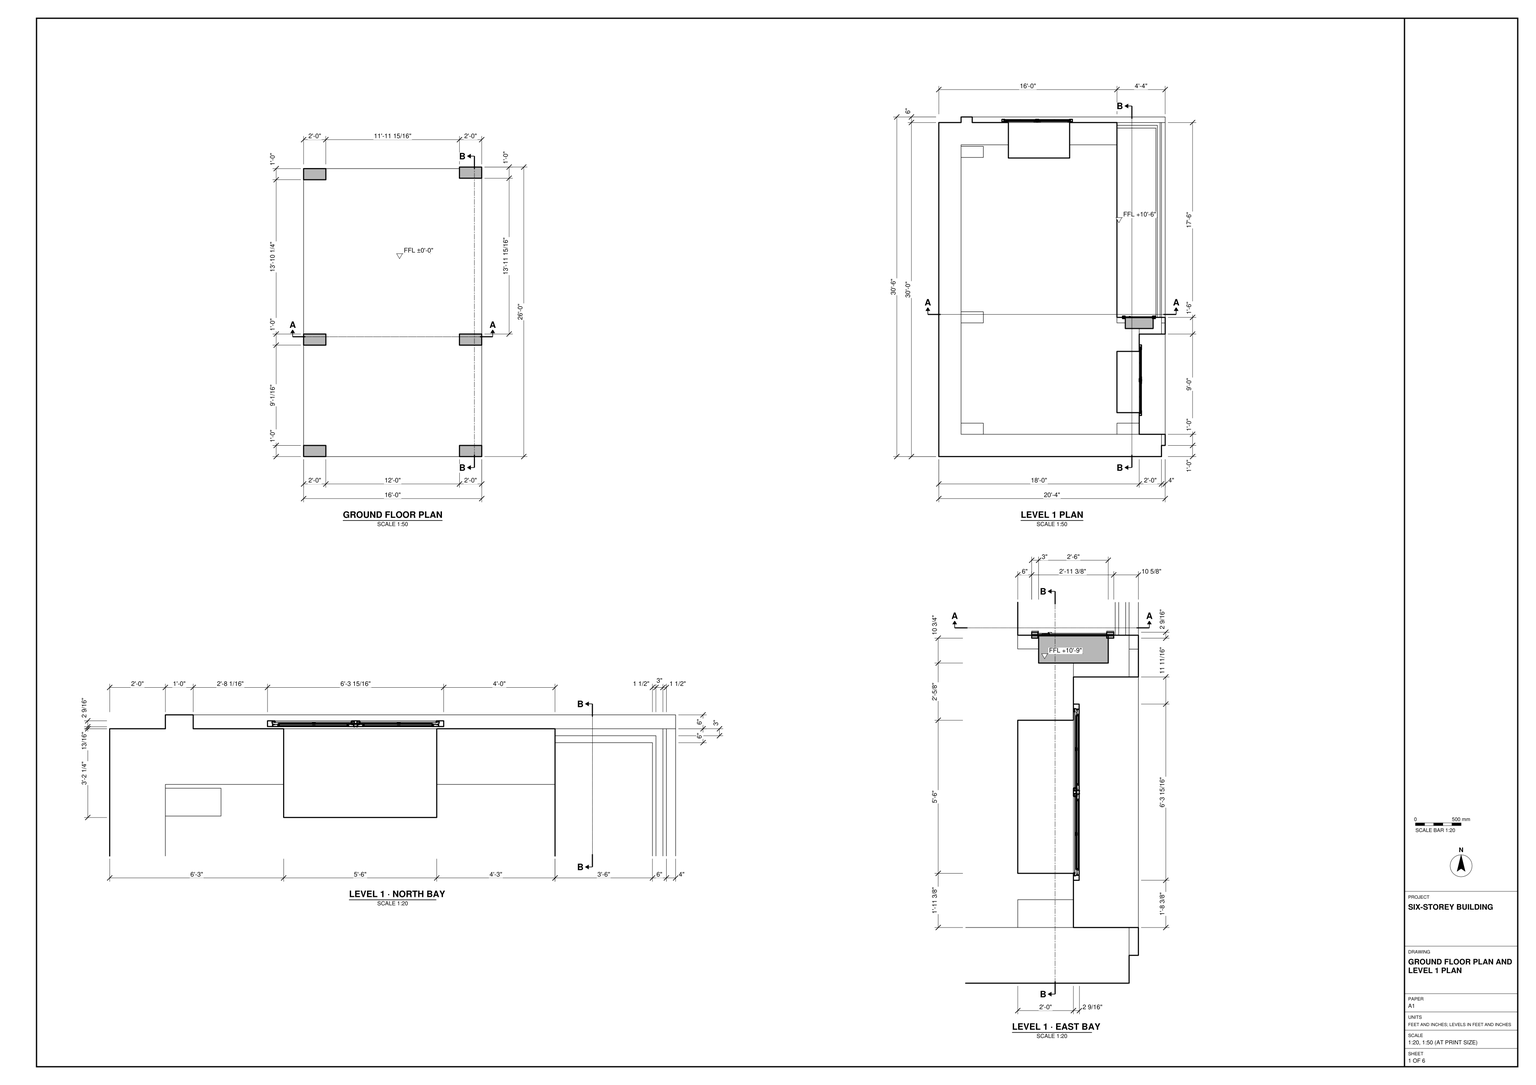
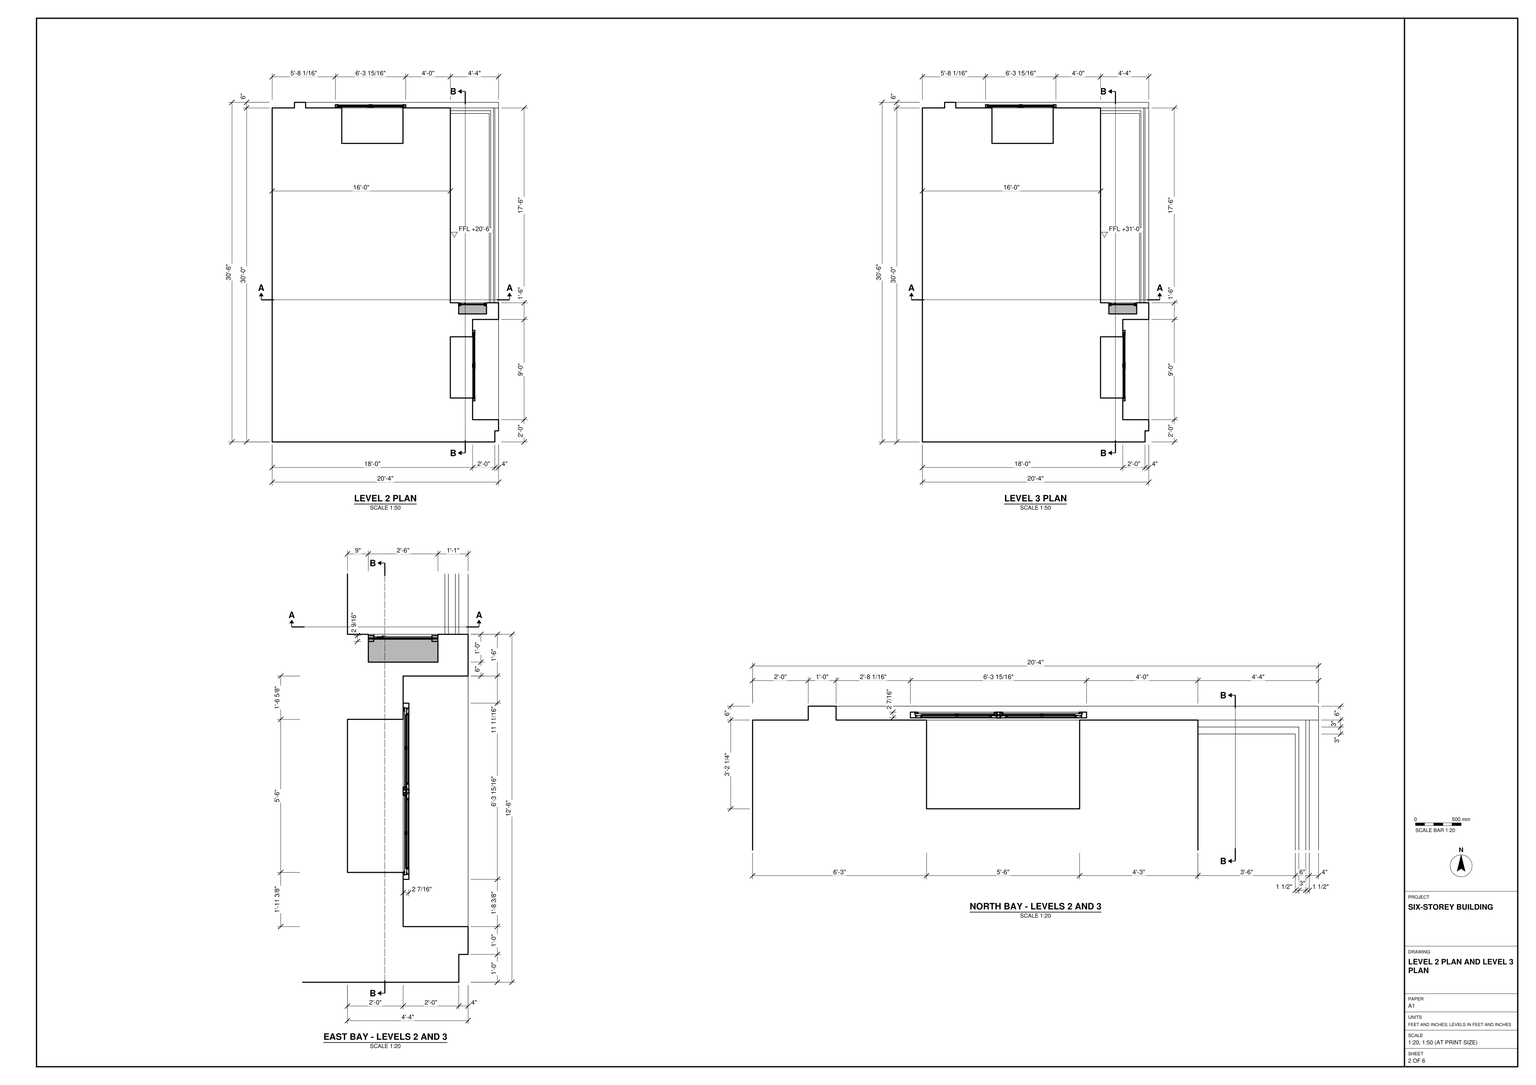
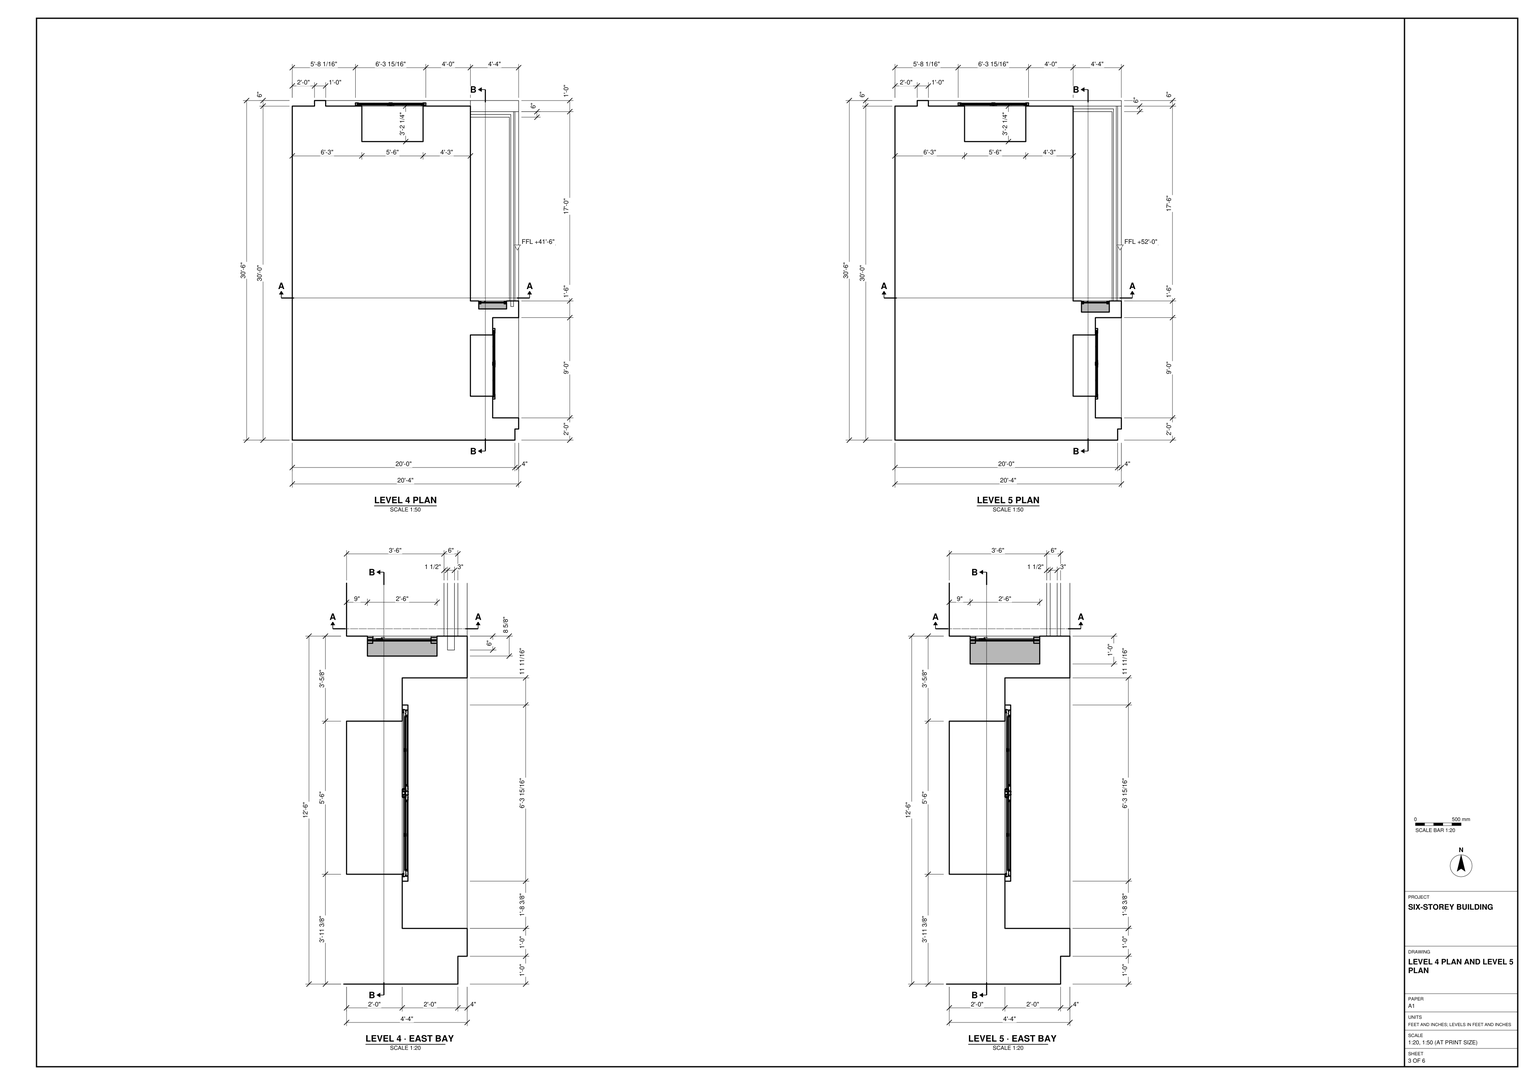
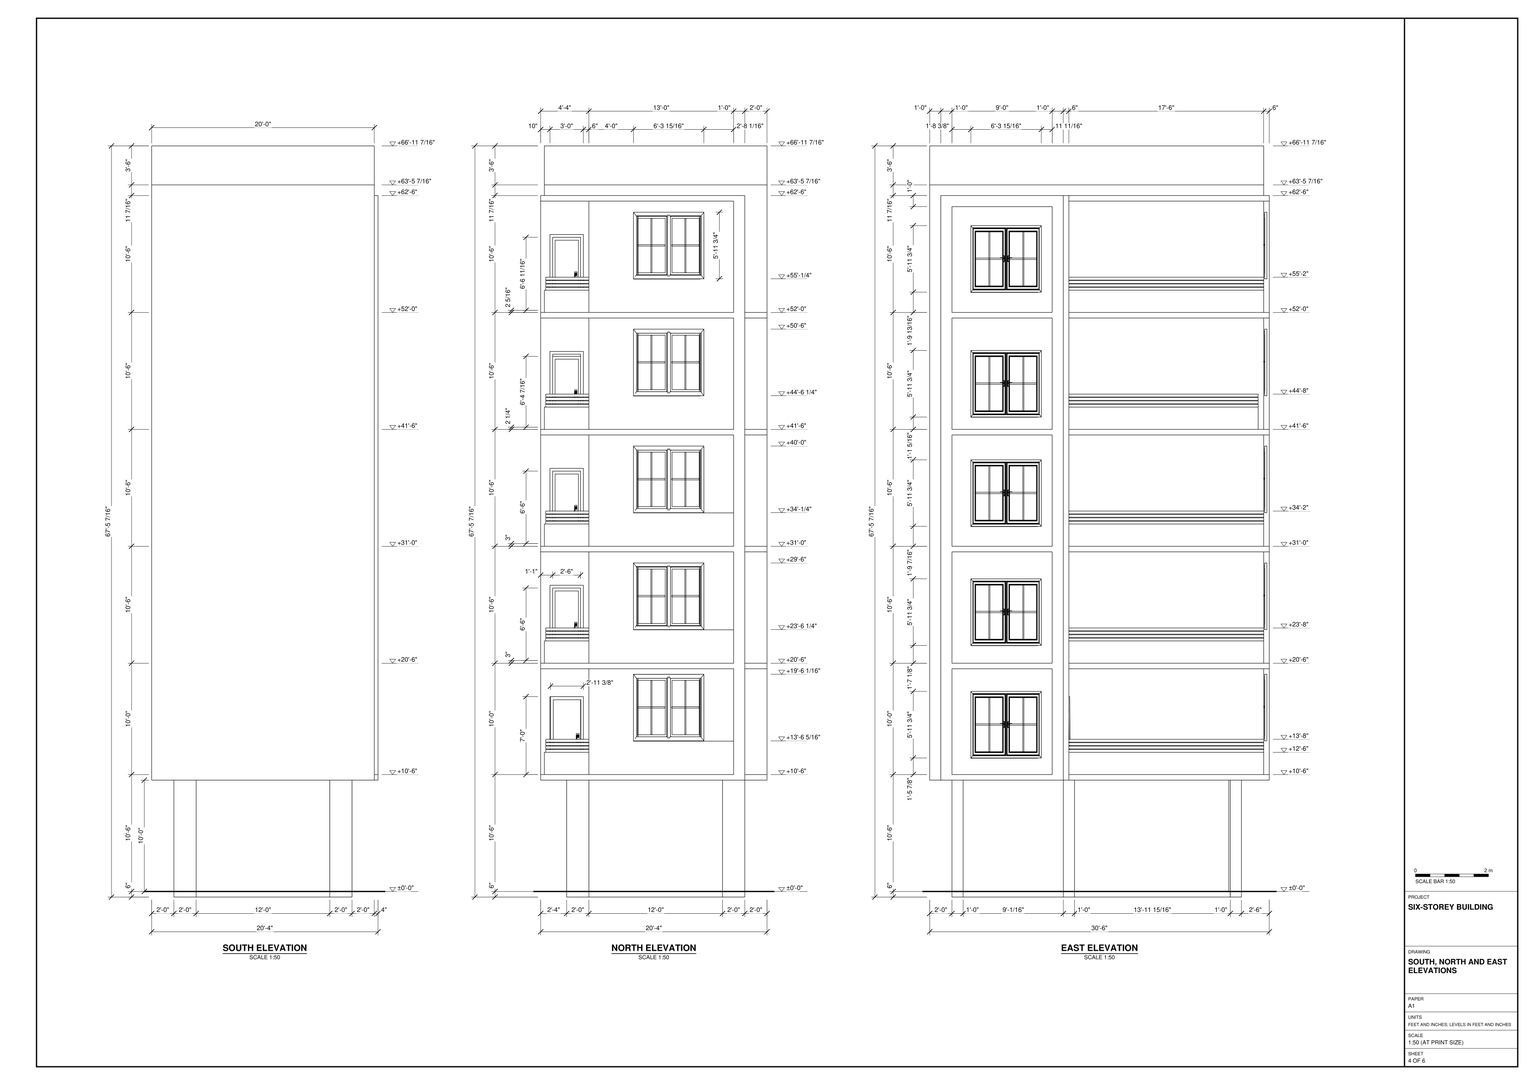
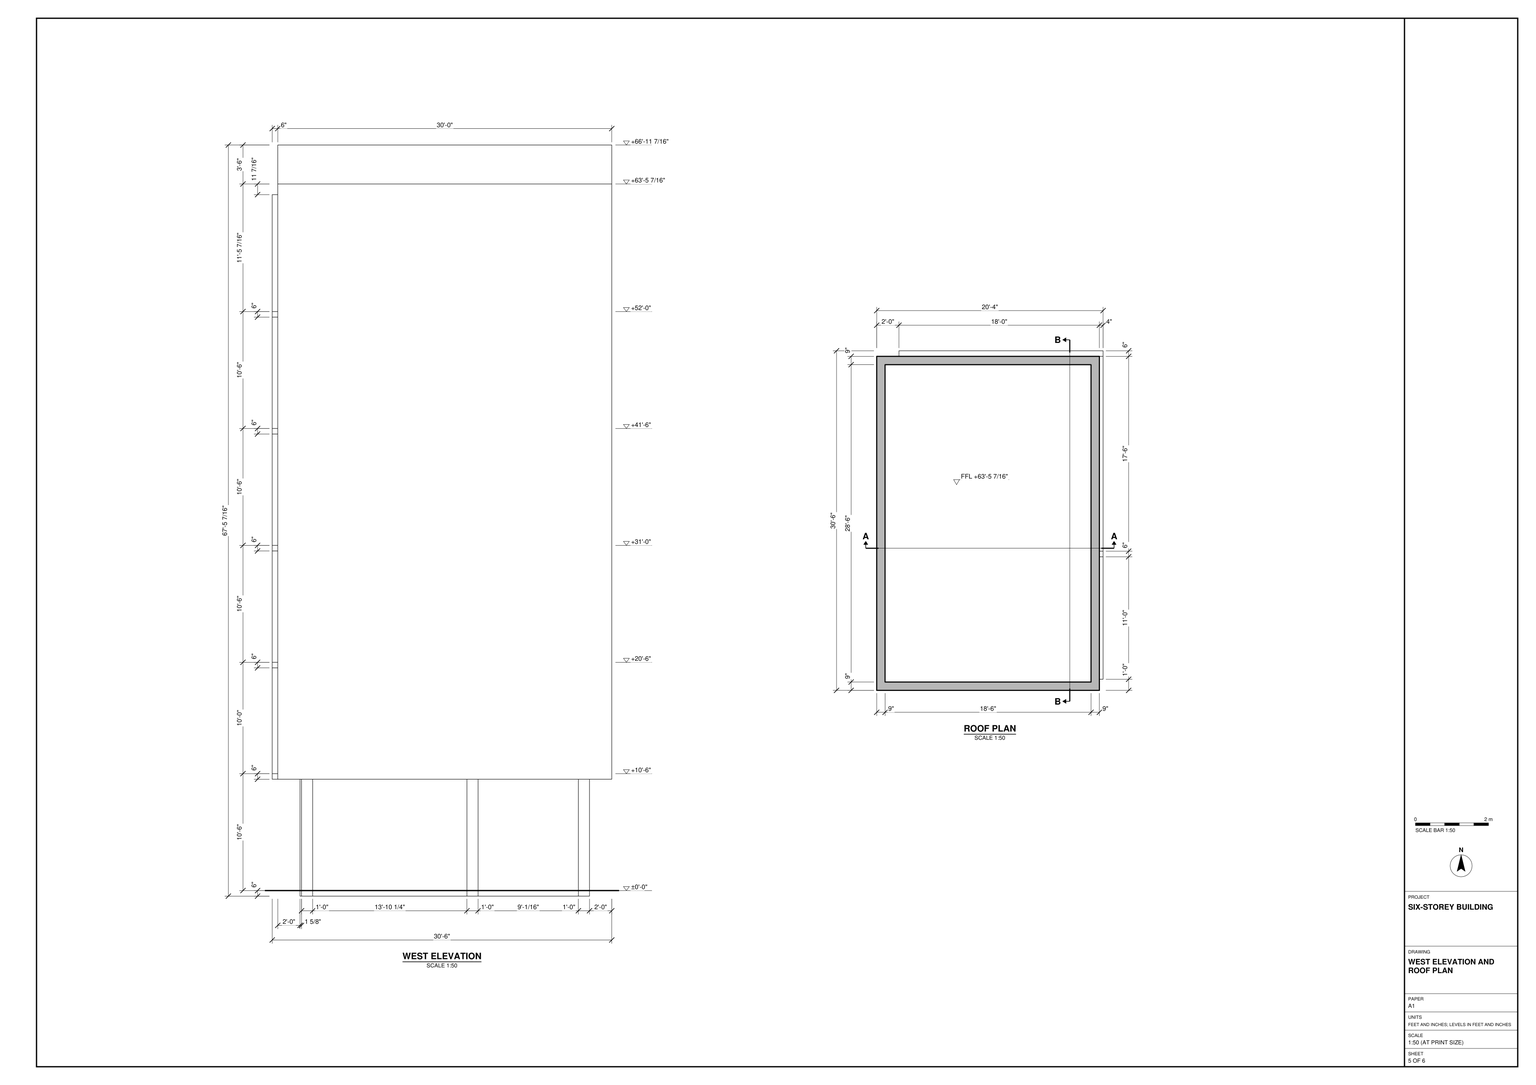
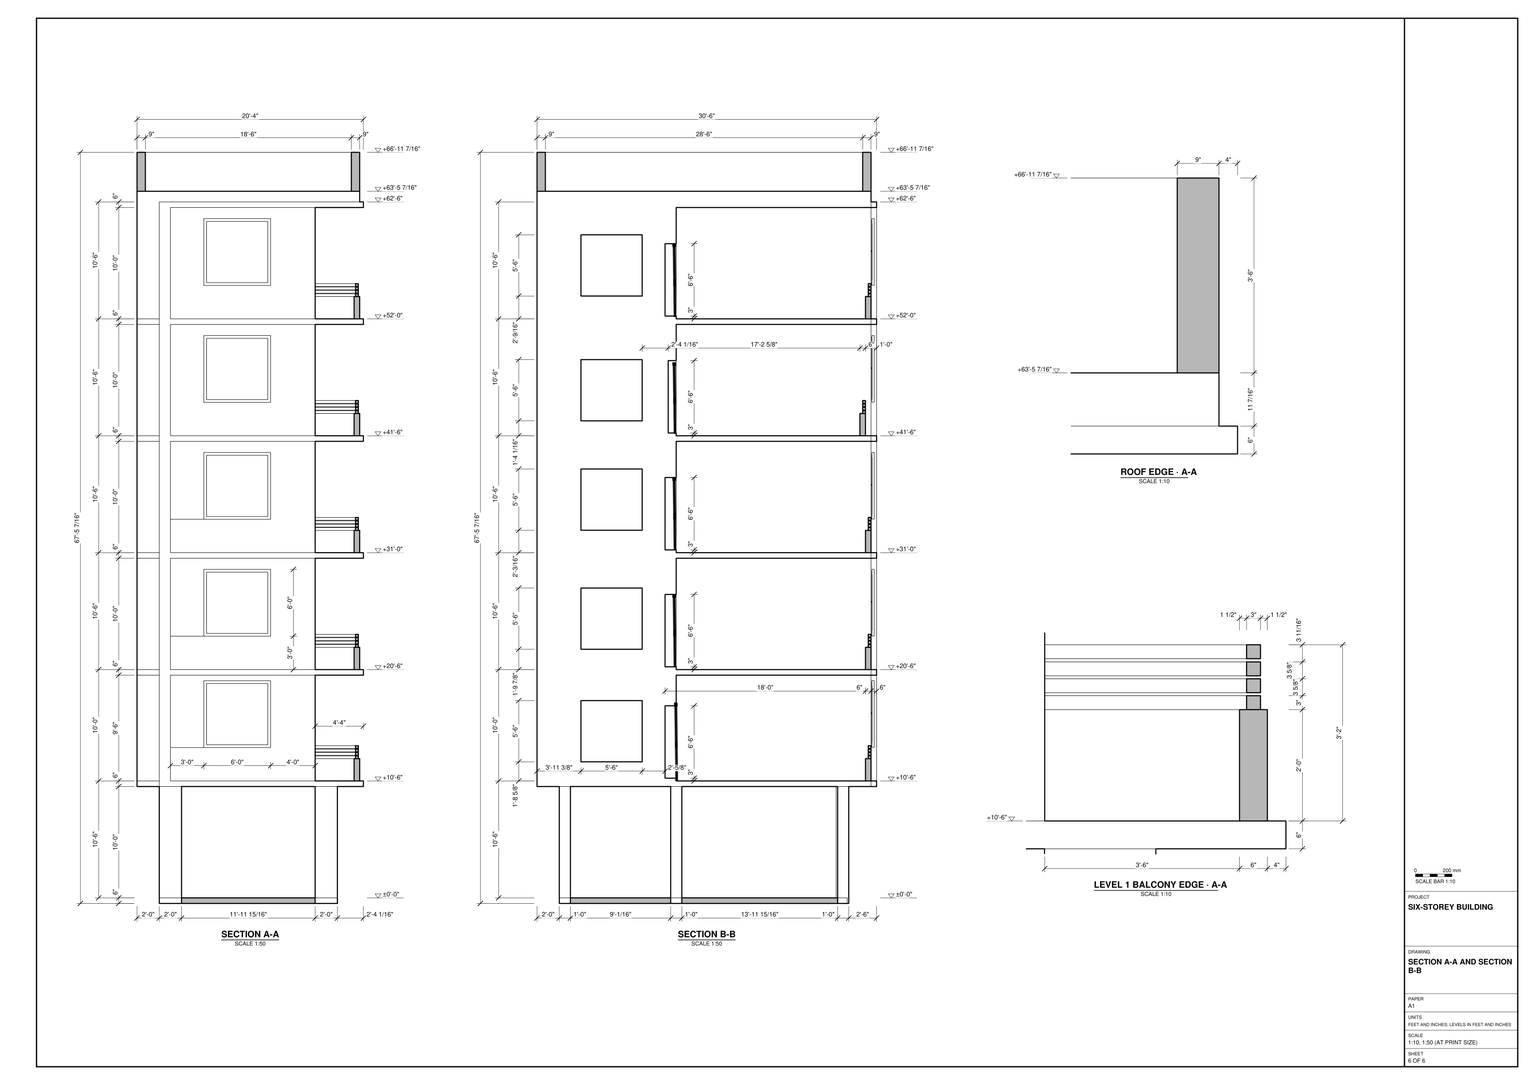
Build the six-storey building in SketchUp from task_files/diagram_01.pdf. Work in feet and inches. The overall size is 20'-4" east to west by 30'-6" north to south, with a total height of 67'-5 7/16". Set the ground floor at ±0'-0" and Levels 1 through 5 at +10'-6", +20'-6", +31'-0", +41'-6" and +52'-0", respectively.

Start with the two rows of rectangular ground-floor columns. Keep the ground storey open and position the upper slabs over the columns using the plans. Model the walls at their drawn thicknesses, the slab edges and the roof profile. On each upper floor, use the enlarged bay plans to locate the north opening, the long narrow bay at the northeast corner and the stepped east wall. Fit the door and window units into the openings, including the opening in the short return at the end of the narrow bay. Follow the detail for each level rather than assuming that every return is identical.

Keep walls, slabs and roof elements in separate groups or components. Group each furniture or joinery piece separately where shown, and use components for repeated parts. Any decor or loose items shown may be represented by suitable library components. Save one SketchUp model as output_files/six_storey_building_with_open_ground_floor.skp.

# SketchUp Ruby script. Lengths in inches.
U = 1.inch
M = Sketchup.active_model
def pt(a) = Geom::Point3d.new(a.map { |v| v * U })
def face(e, loops, mat)
  f = e.add_face(loops[0].map { |a| pt(a) })
  loops[1..].each { |l| e.add_face(l.map { |a| pt(a) }).erase! }
  f.material = f.back_material = mat if mat
  f
end
# faces: each face lists its corners as indices into pts; further lists are holes
def faces(e, pts, list, mat = nil) = list.each { |f| face(e, (f[0].is_a?(Array) ? f : [f]).map { |l| l.map { |i| pts[i] } }, mat) }
# xy, xz, yz: faces in a plane at the given z, y or x. An outline is a flat list of corners, or four numbers for a rectangle; further outlines are holes
def ring(l) = l.size == 4 ? [[l[0], l[1]], [l[2], l[1]], [l[2], l[3]], [l[0], l[3]]] : l.each_slice(2).to_a
def flat(e, list, mat, &to3) = list.each { |f| face(e, (f[0].is_a?(Array) ? f : [f]).map { |l| ring(l).map { |u, v| to3.(u, v) } }, mat) }
def xy(e, z, list, mat = nil) = flat(e, list, mat) { |x, y| [x, y, z] }
def xz(e, y, list, mat = nil) = flat(e, list, mat) { |x, z| [x, y, z] }
def yz(e, x, list, mat = nil) = flat(e, list, mat) { |y, z| [x, y, z] }
def lines(e, pts, list) = list.each { |a, b| e.add_line(pt(pts[a]), pt(pts[b])) }
# prism: a flat outline (further loops are holes) pulled along v
def prism(e, loops, v, mat = nil)
  f = face(e, loops, mat); d = Geom::Vector3d.new(v.map { |x| x * U })
  f.pushpull(f.normal.samedirection?(d) ? d.length : -d.length)
end
def box(e, o, s, mat = nil) = prism(e, [[o, [o[0] + s[0], o[1], o[2]], [o[0] + s[0], o[1] + s[1], o[2]], [o[0], o[1] + s[1], o[2]]]], [0, 0, s[2]], mat)
def at(x, y, z, deg = 0) = Geom::Transformation.translation(pt([x, y, z])) * Geom::Transformation.rotation(ORIGIN, Z_AXIS, deg.degrees)
def axes(o, x, y, z) = Geom::Transformation.new([*x, 0, *y, 0, *z, 0, *pt(o).to_a, 1])
def part(name) = M.definitions.add(name)
# library, detail: a bought-in or finely detailed component or shape, given as its bounding box
def library(name, o, s) = part(name).tap { |d| box(d.entities, o, s) }
def detail(e, o, s) = box(e.add_group.entities, o, s)
def put(e, d, t, mat = nil) = e.add_instance(d, t).tap { |i| i.material = mat if mat }
def group(e, t, mat = nil) = e.add_group.tap { |g| g.transformation = t; g.material = mat if mat }.entities
root = M.entities
M.materials.add("C01_Vanilla_Cream").color = [255, 230, 206]
M.materials.add("Carpet_04_1K").color = [43, 65, 85]
M.materials.add("M00_Soft_Cloud").color = [255, 255, 255]
M.materials.add("[Color_009]1").color = [0, 0, 0]
c1 = library("porta+4",[0.2,-5.42,1.33],[46.55,4.72,83.21])
c2 = library("mesh-163",[-551.08,-704.17,-20.03],[1929.24,1401.85,86.96])
c3 = part("Group11")
put(c3.entities,c2,at(0,0,0))
g1 = group(root,at(0,0,0))
xy(g1,-6,[[24,24,48,36],[[48,24,48,36,24,36,24,144.09,48,144.09,48,156.09,24,156.09,24,322.36,48,322.36,48,334.36,191.96,334.36,191.96,323.92,216,323.92,216,36,192,36,192,24],[191.96,144.09,215.96,156.09]],[192,24,216,36],[24,144.09,48,156.09],[191.96,144.09,215.96,156.09],
  [24,322.36,48,334.36],[191.96,324,215.96,336]])
xy(g1,0,[[[48,24,192,24,192,36,216,36,216,323.92,191.96,323.92,191.96,334.36,48,334.36,48,322.36,24,322.36,24,156.09,48,156.09,48,144.09,24,144.09,24,36,48,36],[191.96,144.09,215.96,156.09]]])
xy(g1,120,[[[0,0,0,360,24,360,24,366,36,366,36,360,240,360,240,0],[24,24,216,336]],[240,12,244,144],[[48,24,48,36,24,36,24,144.09,48,144.09,48,156.09,24,156.09,24,322.36,48,322.36,48,334.36,24,334.36,24,336,191.96,336,191.96,324,215.96,324,215.96,336,216,336,216,36,192,36,192,24],[191.96,144.09,215.96,156.09]],[240,144,244,360],[36,360,244,366]])
xy(g1,126,[[234,150,240,360],[192,354,234,360]])
xy(g1,126,[[216,24,244,132],[192,150,234,354],[240,150,244,360],[36,360,244,366]],"C01_Vanilla_Cream")
xy(g1,129,[[201,138,231,150]])
xy(g1,146.61,[[192,47.35,216,113.35]])
xy(g1,150,[[234,150,235.52,150,235.52,357,192,357,192,354,234,354],[235.52,150,235.52,357,192,357,192,360,238.52,360,238.52,150],[238.52,150,240,360]],"C01_Vanilla_Cream")
xy(g1,153,[[235.52,150,238.52,150,238.52,360,192,360,192,357,235.52,357]],"C01_Vanilla_Cream")
xy(g1,153.65,[[235.52,150,235.52,357,192,357,192,360,238.52,360,238.52,150]],"C01_Vanilla_Cream")
xy(g1,156.65,[[235.52,150,238.52,150,238.52,360,192,360,192,357,235.52,357]],"C01_Vanilla_Cream")
xy(g1,157.28,[[235.52,150,235.52,357,192,357,192,360,238.52,360,238.52,150]],"C01_Vanilla_Cream")
xy(g1,160.28,[[235.52,150,238.52,150,238.52,360,192,360,192,357,235.52,357]],"C01_Vanilla_Cream")
xy(g1,160.98,[[235.52,150,235.52,357,192,357,192,360,238.52,360,238.52,150]],"C01_Vanilla_Cream")
xy(g1,163.98,[[235.52,150,238.52,150,238.52,360,192,360,192,357,235.52,357]],"[Color_009]1")
xy(g1,165,[[75,321.76,141,360]])
xy(g1,207,[[201,138,231,150]])
xy(g1,212.61,[[192,47.35,216,113.35]])
xy(g1,231,[[75,321.76,141,360]])
xy(g1,240,[[216,24,244,132],[36,360,192,366]])
xy(g1,240,[[192,150,244,366]],"C01_Vanilla_Cream")
xy(g1,246,[[234,150,240,360],[192,354,234,360]])
xy(g1,246,[[216,24,244,132],[192,150,234,354],[240,150,244,360],[36,360,244,366]],"C01_Vanilla_Cream")
xy(g1,249,[[201,138,231,150]])
xy(g1,267.9,[[192,47.35,216,113.35]])
xy(g1,270,[[234,150,235.52,150,235.52,357,192,357,192,354,234,354],[235.52,150,235.52,357,192,357,192,360,238.52,360,238.52,150],[238.52,150,240,360]],"C01_Vanilla_Cream")
xy(g1,273,[[235.52,150,238.52,150,238.52,360,192,360,192,357,235.52,357]],"C01_Vanilla_Cream")
xy(g1,273.65,[[235.52,150,235.52,357,192,357,192,360,238.52,360,238.52,150]],"C01_Vanilla_Cream")
xy(g1,276.65,[[235.52,150,238.52,150,238.52,360,192,360,192,357,235.52,357]],"C01_Vanilla_Cream")
xy(g1,277.28,[[235.52,150,235.52,357,192,357,192,360,238.52,360,238.52,150]],"C01_Vanilla_Cream")
xy(g1,280.28,[[235.52,150,238.52,150,238.52,360,192,360,192,357,235.52,357]],"C01_Vanilla_Cream")
xy(g1,280.98,[[235.52,150,235.52,357,192,357,192,360,238.52,360,238.52,150]],"C01_Vanilla_Cream")
xy(g1,283.98,[[235.52,150,238.52,150,238.52,360,192,360,192,357,235.52,357]],"[Color_009]1")
xy(g1,285,[[75,321.76,141,360]])
xy(g1,327,[[201,138,231,150]])
xy(g1,333.9,[[192,47.35,216,113.35]])
xy(g1,351,[[75,321.76,141,360]])
xy(g1,366,[[216,24,244,132],[36,360,192,366]])
xy(g1,366,[[192,150,244,366]],"C01_Vanilla_Cream")
xy(g1,372,[[234,150,240,360],[192,354,234,360]])
xy(g1,372,[[216,24,244,132],[192,150,234,354],[240,150,244,360],[36,360,244,366]],"C01_Vanilla_Cream")
xy(g1,375,[[201,138,231,150]])
xy(g1,396,[[234,150,235.52,150,235.52,357,192,357,192,354,234,354],[235.52,150,235.52,357,192,357,192,360,238.52,360,238.52,150],[238.52,150,240,360]],"C01_Vanilla_Cream")
xy(g1,396.2,[[192,47.35,216,113.35]])
xy(g1,399,[[235.52,150,238.52,150,238.52,360,192,360,192,357,235.52,357]],"C01_Vanilla_Cream")
xy(g1,399.65,[[235.52,150,235.52,357,192,357,192,360,238.52,360,238.52,150]],"C01_Vanilla_Cream")
xy(g1,402.65,[[235.52,150,238.52,150,238.52,360,192,360,192,357,235.52,357]],"C01_Vanilla_Cream")
xy(g1,403.28,[[235.52,150,235.52,357,192,357,192,360,238.52,360,238.52,150]],"C01_Vanilla_Cream")
xy(g1,406.28,[[235.52,150,238.52,150,238.52,360,192,360,192,357,235.52,357]],"C01_Vanilla_Cream")
xy(g1,406.98,[[235.52,150,235.52,357,192,357,192,360,238.52,360,238.52,150]],"C01_Vanilla_Cream")
xy(g1,409.98,[[235.52,150,238.52,150,238.52,360,192,360,192,357,235.52,357]],"[Color_009]1")
xy(g1,411,[[75,321.76,141,360]])
xy(g1,453,[[201,138,231,150]])
xy(g1,462.2,[[192,47.35,216,113.35]])
xy(g1,477,[[75,321.76,141,360]])
xy(g1,492,[[36,360,192,366]])
xy(g1,492,[[216,24,244,132],[192,150,244,366]],"C01_Vanilla_Cream")
xy(g1,498,[[234,150,240,354],[192,348,234,354]])
xy(g1,498,[[216,24,244,132],[192,150,234,348],[240,150,244,354],[192,354,244,366],[36,360,192,366]],"C01_Vanilla_Cream")
xy(g1,501,[[201,141.4,231,150]])
xy(g1,514.07,[[192,47.35,216,113.35]])
xy(g1,522,[[235.52,144,238.52,150],[234,150,235.52,150,235.52,351,192,351,192,348,234,348],[235.52,150,238.52,150,238.52,354,192,354,192,351,235.52,351],[238.52,150,240,354]],"C01_Vanilla_Cream")
xy(g1,525,[[235.52,144,238.52,144,238.52,354,192,354,192,351,235.52,351]],"C01_Vanilla_Cream")
xy(g1,525.6,[[235.52,144,235.52,351,192,351,192,354,238.52,354,238.52,144]],"C01_Vanilla_Cream")
xy(g1,528.65,[[235.52,144,238.52,144,238.52,354,192,354,192,351,235.52,351]],"C01_Vanilla_Cream")
xy(g1,529.28,[[235.52,144,235.52,351,192,351,192,354,238.52,354,238.52,144]],"C01_Vanilla_Cream")
xy(g1,532.28,[[235.52,144,238.52,144,238.52,354,192,354,192,351,235.52,351]],"C01_Vanilla_Cream")
xy(g1,532.98,[[235.52,144,235.52,351,192,351,192,354,238.52,354,238.52,144]],"C01_Vanilla_Cream")
xy(g1,535.98,[[235.52,144,238.52,144,238.52,354,192,354,192,351,235.52,351]],"[Color_009]1")
xy(g1,537,[[75,321.76,141,360]])
xy(g1,579,[[201,141.4,231,150]])
xy(g1,580.07,[[192,47.35,216,113.35]])
xy(g1,603,[[75,321.76,141,360]])
xy(g1,618,[[36,360,192,366]])
xy(g1,618,[[216,24,244,132],[192,150,244,366]],"C01_Vanilla_Cream")
xy(g1,624,[[234,150,240,360],[192,354,234,360]])
xy(g1,624,[[216,24,244,132],[192,150,234,354],[240,150,244,360],[36,360,244,366]],"C01_Vanilla_Cream")
xy(g1,627,[[201,138,231,150]])
xy(g1,648,[[234,150,235.52,150,235.52,357,192,357,192,354,234,354],[235.52,150,238.52,150,238.52,360,192,360,192,357,235.52,357],[238.52,150,240,360]],"C01_Vanilla_Cream")
xy(g1,648.59,[[192,47.35,216,113.35]])
xy(g1,651,[[235.52,150,238.52,150,238.52,360,192,360,192,357,235.52,357]],"[Color_009]1")
xy(g1,651.65,[[235.52,150,235.52,357,192,357,192,360,238.52,360,238.52,150]],"C01_Vanilla_Cream")
xy(g1,654.65,[[235.52,150,238.52,150,238.52,360,192,360,192,357,235.52,357]],"[Color_009]1")
xy(g1,655.28,[[235.52,150,235.52,357,192,357,192,360,238.52,360,238.52,150]],"C01_Vanilla_Cream")
xy(g1,658.28,[[235.52,150,238.52,150,238.52,360,192,360,192,357,235.52,357]],"[Color_009]1")
xy(g1,658.98,[[235.52,150,235.52,357,192,357,192,360,238.52,360,238.52,150]],"C01_Vanilla_Cream")
xy(g1,661.98,[[235.52,150,238.52,150,238.52,360,192,360,192,357,235.52,357]],"[Color_009]1")
xy(g1,663,[[75,321.76,141,360]])
xy(g1,705,[[201,138,231,150]])
xy(g1,714.59,[[192,47.35,216,113.35]])
xy(g1,729,[[75,321.76,141,360]])
xy(g1,738,[[216,24,244,132]])
xy(g1,744,[[36,360,192,366]])
xy(g1,744,[[192,150,244,366]],"C01_Vanilla_Cream")
xy(g1,750,[[240,12,244,144],[240,144,244,150],[240,150,244,360],[24,360,244,366]],"C01_Vanilla_Cream")
xy(g1,761.46,[[9,9,231,351]],"C01_Vanilla_Cream")
xz(g1,0,[[0,120,240,761.46]],"C01_Vanilla_Cream")
xz(g1,12,[[240,120,244,126],[240,126,244,750]])
xz(g1,24,[[24,-6,48,120],[48,-6,192,0],[192,-6,216,120]])
xz(g1,24,[[216,126,244,240],[216,246,244,366],[216,372,244,492],[216,498,244,618],[216,624,244,738]],"C01_Vanilla_Cream")
xz(g1,36,[[24,-6,48,0],[192,-6,216,0],[24,0,48,120],[192,0,216,120]])
xz(g1,47.35,[[192,146.61,216,212.61],[192,267.9,216,333.9],[192,396.2,216,462.2],[192,514.07,216,580.07],[192,648.59,216,714.59]])
xz(g1,113.35,[[192,146.61,216,212.61],[192,267.9,216,333.9],[192,396.2,216,462.2],[192,514.07,216,580.07],[192,648.59,216,714.59]])
xz(g1,132,[[216,126,244,240],[216,246,244,366],[216,372,244,492],[216,498,244,618],[216,624,244,738]],"C01_Vanilla_Cream")
xz(g1,138,[[201,129,231,207],[201,249,231,327],[201,375,231,453],[201,627,231,705]])
xz(g1,141.4,[[201,501,231,579]])
xz(g1,144,[[235.52,522,238.52,525],[235.52,525.6,238.52,528.65],[235.52,529.28,238.52,532.28],[235.52,532.98,238.52,535.98]],"C01_Vanilla_Cream")
xz(g1,144.09,[[24,-6,48,0],[191.96,-6,215.96,0],[24,0,48,120],[191.96,0,215.96,120]])
xz(g1,150,[[[198,126,234,210],[201,129,231,207]],[234,126,240,150],[[198,246,234,330],[201,249,231,327]],[234,246,240,270],[[198,372,234,456],[201,375,231,453]],
  [234,372,240,396],[[198,498,234,582],[201,501,231,579]],[234,498,240,522],[[198,624,234,708],[201,627,231,705]],[234,624,240,648]])
xz(g1,150,[[192,126,192,240,244,240,244,126,240,126,240,150,238.52,150,238.52,153,235.52,153,235.52,150,234,150,234,210,198,210,198,126],[235.52,150,238.52,153],[235.52,153.65,238.52,156.65],[235.52,157.28,238.52,160.28],[235.52,160.98,238.52,163.98],
  [192,246,192,366,244,366,244,246,240,246,240,270,238.52,270,238.52,273,235.52,273,235.52,270,234,270,234,330,198,330,198,246],[235.52,270,238.52,273],[235.52,273.65,238.52,276.65],[235.52,277.28,238.52,280.28],[235.52,280.98,238.52,283.98],
  [192,372,192,492,244,492,244,372,240,372,240,396,238.52,396,238.52,399,235.52,399,235.52,396,234,396,234,456,198,456,198,372],[235.52,396,238.52,399],[235.52,399.65,238.52,402.65],[235.52,403.28,238.52,406.28],[235.52,406.98,238.52,409.98],
  [192,498,192,618,244,618,244,498,240,498,240,522,234,522,234,582,198,582,198,498],[[192,624,192,744,244,744,244,624,240,624,240,648,238.52,648,238.52,651,235.52,651,235.52,648,234,648,234,708,198,708,198,624],[235.52,651.65,238.52,654.65],[235.52,655.28,238.52,658.28],[235.52,658.98,238.52,661.98]]],"C01_Vanilla_Cream")
xz(g1,156.09,[[24,-6,48,0],[191.96,-6,215.96,0],[24,0,48,120],[191.96,0,215.96,120]])
xz(g1,321.76,[[75,165,141,231],[75,285,141,351],[75,411,141,477],[75,537,141,603],[75,663,141,729]])
xz(g1,322.36,[[24,-6,48,0],[24,0,48,120]])
xz(g1,323.92,[[191.96,-6,216,0]])
xz(g1,324,[[191.96,-6,215.96,0],[191.96,0,215.96,120]])
xz(g1,334.36,[[24,-6,48,120],[48,-6,191.96,0]])
xz(g1,336,[[191.96,-6,215.96,120]])
xz(g1,348,[[192,498,234,522]],"C01_Vanilla_Cream")
xz(g1,351,[[192,522,235.52,525],[192,525.6,235.52,528.65],[192,529.28,235.52,532.28],[192,532.98,235.52,535.98]],"C01_Vanilla_Cream")
xz(g1,354,[[192,126,234,150],[192,246,234,270],[192,372,234,396],[192,498,240,522],[192,624,234,648]],"C01_Vanilla_Cream")
xz(g1,354,[[192,522,238.52,525],[192,525.6,238.52,528.65],[192,529.28,238.52,532.28],[192,532.98,238.52,535.98]],"[Color_009]1")
xz(g1,357,[[192,150,235.52,153],[192,153.65,235.52,156.65],[192,157.28,235.52,160.28],[192,160.98,235.52,163.98],[192,270,235.52,273],
  [192,273.65,235.52,276.65],[192,277.28,235.52,280.28],[192,280.98,235.52,283.98],[192,396,235.52,399],[192,399.65,235.52,402.65],
  [192,403.28,235.52,406.28],[192,406.98,235.52,409.98],[192,648,235.52,651],[192,651.65,235.52,654.65],[192,655.28,235.52,658.28],
  [192,658.98,235.52,661.98]],"C01_Vanilla_Cream")
xz(g1,360,[[[72,162,144,234],[75,165,141,231]],[[72,282,144,354],[75,285,141,351]],[[72,408,144,480],[75,411,141,477]],[[72,534,144,606],[75,537,141,603]],[[72,660,144,732],[75,663,141,729]]])
xz(g1,360,[[0,120,24,126],[0,126,24,240],[36,126,36,162,144,162,144,234,72,234,72,162,36,162,36,240,192,240,192,126],[192,126,240,150],[0,240,24,246],
  [0,246,24,366],[36,246,36,282,144,282,144,354,72,354,72,282,36,282,36,366,192,366,192,246],[192,246,240,270],[0,366,24,372],[0,372,24,492],
  [36,372,36,408,144,408,144,480,72,480,72,408,36,408,36,492,192,492,192,372],[192,372,240,396],[0,492,24,498],[0,498,24,618],[[36,498,192,618],[72,534,144,606]],
  [0,618,24,624],[0,624,0,761.46,240,761.46,240,750,24,750,24,624],[[36,624,192,744],[72,660,144,732]],[192,624,240,648]],"C01_Vanilla_Cream")
xz(g1,360,[[192,150,238.52,153],[192,153.65,238.52,156.65],[192,157.28,238.52,160.28],[192,160.98,238.52,163.98],[192,270,238.52,273],
  [192,273.65,238.52,276.65],[192,277.28,238.52,280.28],[192,280.98,238.52,283.98],[192,396,238.52,399],[192,399.65,238.52,402.65],
  [192,403.28,238.52,406.28],[192,406.98,238.52,409.98],[192,648,238.52,651],[192,651.65,238.52,654.65],[192,655.28,238.52,658.28],
  [192,658.98,238.52,661.98]],"[Color_009]1")
xz(g1,366,[[24,120,24,750,244,750,244,744,36,744,36,624,244,624,244,618,36,618,36,498,244,498,244,492,36,492,36,372,244,372,244,366,36,366,36,246,244,246,244,240,36,240,36,126,244,126,244,120]],"C01_Vanilla_Cream")
yz(g1,0,[[0,120,360,761.46]],"C01_Vanilla_Cream")
yz(g1,24,[[24,-6,36,120],[36,-6,144.09,0],[144.09,-6,156.09,120],[156.09,-6,322.36,0],[322.36,-6,334.36,120]])
yz(g1,24,[[360,120,366,126],[360,126,366,240],[360,240,366,246],[360,246,366,366],[360,366,366,372],
  [360,372,366,492],[360,492,366,498],[360,498,366,618],[360,618,366,624],[360,624,366,750]],"C01_Vanilla_Cream")
yz(g1,36,[[360,126,366,240],[360,246,366,366],[360,372,366,492],[360,498,366,618],[360,624,366,744]],"C01_Vanilla_Cream")
yz(g1,48,[[24,-6,36,0],[144.09,-6,156.09,0],[322.36,-6,334.36,0],[24,0,36,120],[144.09,0,156.09,120],
  [322.36,0,334.36,120]])
yz(g1,75,[[321.76,165,360,231],[321.76,285,360,351],[321.76,411,360,477],[321.76,537,360,603],[321.76,663,360,729]])
yz(g1,141,[[321.76,165,360,231],[321.76,285,360,351],[321.76,411,360,477],[321.76,537,360,603],[321.76,663,360,729]])
yz(g1,191.96,[[144.09,-6,156.09,0],[323.92,-6,324,0],[324,-6,334.36,0],[334.36,-6,334.36,0,324,0,324,120,336,120,336,-6],[144.09,0,156.09,120]])
yz(g1,192,[[24,-6,36,0],[24,0,36,120],[354,126,360,150],[47.35,146.61,113.35,212.61],[354,246,360,270],
  [47.35,267.9,113.35,333.9],[354,372,360,396],[47.35,396.2,113.35,462.2],[348,498,354,522],[47.35,514.07,113.35,580.07],
  [354,624,360,648],[47.35,648.59,113.35,714.59]])
yz(g1,192,[[150,126,354,126,354,150,357,150,357,153,360,153,360,153.65,357,153.65,357,156.65,360,156.65,360,157.28,357,157.28,357,160.28,360,160.28,360,160.98,357,160.98,357,163.98,360,163.98,360,240,150,240],[357,150,360,153],[357,153.65,360,156.65],[357,157.28,360,160.28],[357,160.98,360,163.98],
  [150,246,354,246,354,270,357,270,357,273,360,273,360,273.65,357,273.65,357,276.65,360,276.65,360,277.28,357,277.28,357,280.28,360,280.28,360,280.98,357,280.98,357,283.98,360,283.98,360,366,150,366],[357,270,360,273],[357,273.65,360,276.65],[357,277.28,360,280.28],[357,280.98,360,283.98],
  [150,372,354,372,354,396,357,396,357,399,360,399,360,399.65,357,399.65,357,402.65,360,402.65,360,403.28,357,403.28,357,406.28,360,406.28,360,406.98,357,406.98,357,409.98,360,409.98,360,492,150,492],[357,396,360,399],[357,399.65,360,402.65],[357,403.28,360,406.28],[357,406.98,360,409.98],
  [150,498,348,498,348,522,351,522,351,525,354,525,354,498,360,498,360,618,150,618],[351,522,354,525],[351,525.6,354,528.65],[351,529.28,354,532.28],[351,532.98,354,535.98],
  [150,624,354,624,354,648,357,648,357,651,360,651,360,651.65,357,651.65,357,654.65,360,654.65,360,655.28,357,655.28,357,658.28,360,658.28,360,658.98,357,658.98,357,661.98,360,661.98,360,744,150,744]],"C01_Vanilla_Cream")
yz(g1,201,[[138,129,150,207],[138,249,150,327],[138,375,150,453],[141.4,501,150,579],[138,627,150,705]])
yz(g1,215.96,[[144.09,-6,156.09,0],[324,-6,336,120],[144.09,0,156.09,120]])
yz(g1,216,[[24,-6,36,120],[36,-6,323.92,0],[[44.35,143.61,116.35,215.61],[47.35,146.61,113.35,212.61]],[[44.35,264.9,116.35,336.9],[47.35,267.9,113.35,333.9]],[[44.35,393.2,116.35,465.2],[47.35,396.2,113.35,462.2]],
  [[44.35,511.07,116.35,583.07],[47.35,514.07,113.35,580.07]],[[44.35,645.59,116.35,717.59],[47.35,648.59,113.35,714.59]]])
yz(g1,216,[[[24,126,132,240],[44.35,143.61,116.35,215.61]],[[24,246,132,366],[44.35,264.9,116.35,336.9]],[[24,372,132,492],[44.35,393.2,116.35,465.2]],[[24,498,132,618],[44.35,511.07,116.35,583.07]],[[24,624,132,738],[44.35,645.59,116.35,717.59]]],"C01_Vanilla_Cream")
yz(g1,231,[[138,129,150,150],[138,150,150,207],[138,249,150,270],[138,270,150,327],[138,375,150,396],
  [138,396,150,453],[141.4,501,150,522],[141.4,522,150,579],[138,627,150,648],[138,648,150,705]])
yz(g1,234,[[150,126,354,150],[150,246,354,270],[150,372,354,396],[150,498,348,522],[150,624,354,648]])
yz(g1,235.52,[[150,150,357,153],[150,153.65,357,156.65],[150,157.28,357,160.28],[150,160.98,357,163.98],[150,270,357,273],
  [150,273.65,357,276.65],[150,277.28,357,280.28],[150,280.98,357,283.98],[150,396,357,399],[150,399.65,357,402.65],
  [150,403.28,357,406.28],[150,406.98,357,409.98],[144,522,351,525],[144,525.6,351,528.65],[144,529.28,351,532.28],
  [144,532.98,351,535.98],[150,648,357,651],[150,651.65,357,654.65],[150,655.28,357,658.28],[150,658.98,357,661.98]],"C01_Vanilla_Cream")
yz(g1,238.52,[[150,150,360,153],[150,153.65,360,156.65],[150,157.28,360,160.28],[150,160.98,360,163.98],[150,270,360,273],
  [150,273.65,360,276.65],[150,277.28,360,280.28],[150,280.98,360,283.98],[150,396,360,399],[150,399.65,360,402.65],
  [150,403.28,360,406.28],[150,406.98,360,409.98],[144,522,354,525],[144,525.6,354,528.65],[144,529.28,354,532.28],
  [144,532.98,354,535.98],[150,648,360,651],[150,651.65,360,654.65],[150,655.28,360,658.28],[150,658.98,360,661.98]],"[Color_009]1")
yz(g1,240,[[0,120,12,120,12,750,360,750,360,761.46,0,761.46],[150,126,360,150],[150,246,360,270],[150,372,360,396],[150,498,354,522],
  [150,624,360,648]],"C01_Vanilla_Cream")
yz(g1,244,[[150,120,366,126],[150,240,366,246],[150,366,366,372],[150,492,366,498],[150,618,366,624],
  [150,744,366,750]],"C01_Vanilla_Cream")
yz(g1,244,[[144,120,150,750]],"Carpet_04_1K")
yz(g1,244,[[[12,120,144,750],[24,498,132,618],[24,246,132,366],[24,372,132,492],[24,126,132,240],[24,624,132,738]]],"M00_Soft_Cloud")
p = [[235.52,357,655.28],[235.52,357,654.65],[235.52,357,651.65],[235.52,357,651],[216,334.36,0],[215.96,334.36,0]]
lines(g1,p,[[0,1],[2,3],[4,5]])
put(g1,c1,axes([197.85,153.64,124.61],[0.76,0,0],[0,1,0],[0,0,1.01005]))
put(g1,c1,axes([200.87,151.84,247.71],[0.64449,0,0],[0,1,0],[0,0,0.93794]))
put(g1,c1,axes([200.87,151.84,373.71],[0.64449,0,0],[0,1,0],[0,0,0.93794]))
put(g1,c1,axes([200.87,151.85,499.04],[0.64449,0,0],[0,1,0],[0,0,0.91918]))
put(g1,c1,axes([200.87,151.85,625.02],[0.64449,0,0],[0,1,0],[0,0,0.94616]))
put(g1,c3,axes([89.74,362.63,696.29],[0.03937,0,0],[0,0,0.05118],[0,-0.03937,0]))
put(g1,c3,axes([89.74,362.63,570.29],[0.03937,0,0],[0,0,0.05118],[0,-0.03937,0]))
put(g1,c3,axes([89.74,362.63,444.29],[0.03937,0,0],[0,0,0.05118],[0,-0.03937,0]))
put(g1,c3,axes([89.74,362.63,318.29],[0.03937,0,0],[0,0,0.05118],[0,-0.03937,0]))
put(g1,c3,axes([89.74,362.63,198.38],[0.03937,0,0],[0,0,0.05118],[0,-0.03937,0]))
put(g1,c3,axes([216.79,66.04,179.9],[0,0.03937,0],[0,0,0.05118],[0.03937,0,0]))
put(g1,c3,axes([216.79,66.04,301.1875],[0,0.03937,0],[0,0,0.05118],[0.03937,0,0]))
put(g1,c3,axes([216.79,66.04,429.49],[0,0.03937,0],[0,0,0.05118],[0.03937,0,0]))
put(g1,c3,axes([216.79,66.04,547.36],[0,0.03937,0],[0,0,0.05118],[0.03937,0,0]))
put(g1,c3,axes([216.79,66.04,681.88],[0,0.03937,0],[0,0,0.05118],[0.03937,0,0]))
g2 = group(g1,at(0,0,761.46),"Carpet_04_1K")
prism(g2,[[[0,0,0],[0,360,0],[240,360,0],[240,0,0]],[[9,351,0],[9,9,0],[231,9,0],[231,351,0]]],[0,0,42])
